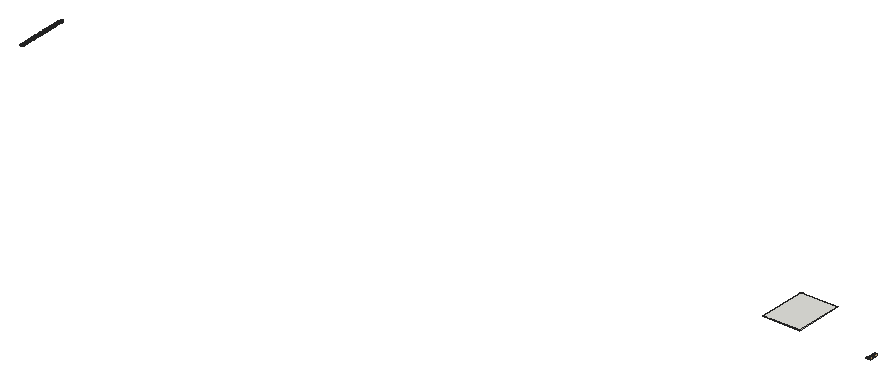
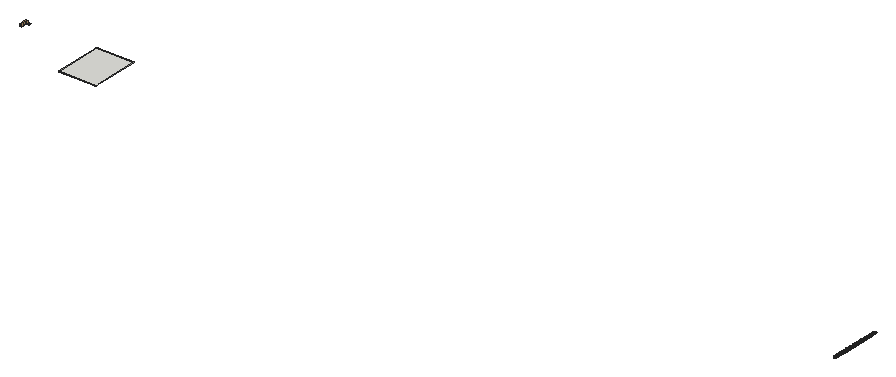
# SketchUp Ruby script. Lengths in inches.
U = 1.inch
M = Sketchup.active_model
def pt(a) = Geom::Point3d.new(a.map { |v| v * U })
def face(e, loops, mat)
  f = e.add_face(loops[0].map { |a| pt(a) })
  loops[1..].each { |l| e.add_face(l.map { |a| pt(a) }).erase! }
  f.material = f.back_material = mat if mat
  f
end
# faces: each face lists its corners as indices into pts; further lists are holes
def faces(e, pts, list, mat = nil) = list.each { |f| face(e, (f[0].is_a?(Array) ? f : [f]).map { |l| l.map { |i| pts[i] } }, mat) }
# xy, xz, yz: faces in a plane at the given z, y or x. An outline is a flat list of corners, or four numbers for a rectangle; further outlines are holes
def ring(l) = l.size == 4 ? [[l[0], l[1]], [l[2], l[1]], [l[2], l[3]], [l[0], l[3]]] : l.each_slice(2).to_a
def flat(e, list, mat, &to3) = list.each { |f| face(e, (f[0].is_a?(Array) ? f : [f]).map { |l| ring(l).map { |u, v| to3.(u, v) } }, mat) }
def xy(e, z, list, mat = nil) = flat(e, list, mat) { |x, y| [x, y, z] }
def xz(e, y, list, mat = nil) = flat(e, list, mat) { |x, z| [x, y, z] }
def yz(e, x, list, mat = nil) = flat(e, list, mat) { |y, z| [x, y, z] }
def lines(e, pts, list) = list.each { |a, b| e.add_line(pt(pts[a]), pt(pts[b])) }
# prism: a flat outline (further loops are holes) pulled along v
def prism(e, loops, v, mat = nil)
  f = face(e, loops, mat); d = Geom::Vector3d.new(v.map { |x| x * U })
  f.pushpull(f.normal.samedirection?(d) ? d.length : -d.length)
end
def box(e, o, s, mat = nil) = prism(e, [[o, [o[0] + s[0], o[1], o[2]], [o[0] + s[0], o[1] + s[1], o[2]], [o[0], o[1] + s[1], o[2]]]], [0, 0, s[2]], mat)
def at(x, y, z, deg = 0) = Geom::Transformation.translation(pt([x, y, z])) * Geom::Transformation.rotation(ORIGIN, Z_AXIS, deg.degrees)
def axes(o, x, y, z) = Geom::Transformation.new([*x, 0, *y, 0, *z, 0, *pt(o).to_a, 1])
def part(name) = M.definitions.add(name)
# library, detail: a bought-in or finely detailed component or shape, given as its bounding box
def library(name, o, s) = part(name).tap { |d| box(d.entities, o, s) }
def detail(e, o, s) = box(e.add_group.entities, o, s)
def put(e, d, t, mat = nil) = e.add_instance(d, t).tap { |i| i.material = mat if mat }
def group(e, t, mat = nil) = e.add_group.tap { |g| g.transformation = t; g.material = mat if mat }.entities
root = M.entities
M.materials.add("Material10").color = [48, 90, 38]
M.materials.add("Material11").color = [68, 110, 48]
M.materials.add("Material12").color = [48, 90, 48]
M.materials.add("Material13").color = [58, 110, 58]
M.materials.add("Material14").color = [58, 90, 38]
M.materials.add("Material15").color = [68, 100, 58]
M.materials.add("Material16").color = [48, 100, 38]
M.materials.add("Material9").color = [68, 110, 58]
c1 = part("grass00")
p = [[-0.6875,0.15,0],[-0.56,0.08,5.52],[-0.04,0.03,2.76],[0.48,-0.02,0],[0.35,-0.02,5.52],[-0.1,-0.14,5.52],
  [-0.12,0.65,8.37],[-0.42,0.65,8.37]]
faces(c1.entities,p,[[0,1,2,3],[3,2,4],[1,5,2],[5,4,2],[1,6,5],[4,5,6],[7,6,1]])
c2 = part("Group16\#1")
put(c2.entities,c1,axes([1.44,-0.61,-0.01],[0.05352,0.12609,0],[-0.10704,0.04543,0.07239],[0.06664,-0.02828,0.11628]),"Material12")
put(c2.entities,c1,axes([0.76,-0.15,-0.01],[0.04676,0.24062,0],[-0.23162,0.04501,0.06642],[0.0652,-0.01267,0.23595]),"Material9")
put(c2.entities,c1,axes([0.79,0.01,-0.01],[-0.00606,0.34651,0],[-0.34381,-0.00602,0.0432],[0.04319,0.00076,0.34386]))
put(c2.entities,c1,axes([1,0.23,-0.01],[-0.07192,0.31144,0],[-0.28722,-0.06632,0.1236],[0.12043,0.02781,0.29478]),"Material11")
put(c2.entities,c1,axes([1.66,0.77,-0.01],[-0.13828,0.29651,0],[-0.21551,-0.1005,0.22471],[0.20365,0.09498,0.23779]),"Material16")
put(c2.entities,c1,axes([0.6875,0.52,-0.01],[-0.18126,0.24051,0],[-0.22746,-0.17142,0.09788],[0.07817,0.05891,0.28481]),"Material11")
put(c2.entities,c1,axes([0.68,0.78,-0.01],[-0.215,0.18688,0],[-0.12385,-0.14248,0.21334],[0.13995,0.16101,0.18878]),"Material9")
put(c2.entities,c1,axes([0.56,1,-0.01],[-0.13756,0.07624,0],[-0.06159,-0.11112,0.0927],[0.04494,0.08108,0.12705]),"Material11")
put(c2.entities,c1,axes([0.2,0.64,-0.01],[-0.23729,0.07254,0],[-0.05711,-0.18681,0.153],[0.04473,0.14632,0.19535]),"Material16")
put(c2.entities,c1,axes([0.0625,0.72,-0.01],[-0.28874,0.02525,0],[-0.02179,-0.24916,0.14647],[0.01276,0.14591,0.25012]),"Material9")
put(c2.entities,c1,axes([-0.08,0.62,-0.01],[-0.34089,-0.04187,0],[0.03255,-0.26504,0.216],[-0.02633,0.21439,0.26703]),"Material16")
put(c2.entities,c1,axes([-0.34,0.98,-0.01],[-0.14314,-0.0493,0],[0.04397,-0.12769,0.06843],[-0.02228,0.0647,0.13505]),"Material16")
put(c2.entities,c1,axes([-0.87,1.45,-0.01],[-0.23488,-0.14114,0],[0.13761,-0.22901,0.06087],[-0.03135,0.05217,0.26717]))
put(c2.entities,c1,axes([-0.72,0.77,-0.01],[-0.14208,-0.13251,0],[0.07209,-0.0773,0.16301],[-0.11118,0.11922,0.1057]),"Material16")
put(c2.entities,c1,axes([-0.62,0.43,-0.01],[-0.14845,-0.21203,0],[0.18654,-0.13061,0.12304],[-0.10079,0.07057,0.22772]),"Material9")
put(c2.entities,c1,axes([-0.68,0.29,-0.01],[-0.13639,-0.32136,0],[0.31723,-0.13464,0.05579],[-0.05136,0.0218,0.34462]),"Material10")
put(c2.entities,c1,axes([-0.64,0.125,-0.01],[-0.0458,-0.23569,0],[0.22124,-0.043,0.08276],[-0.08124,0.01579,0.22538]),"Material13")
put(c2.entities,c1,axes([-1.6,-0.03,-0.01],[0.00576,-0.32897,0],[0.27526,0.00482,0.18018],[-0.18015,-0.00315,0.2753]),"Material11")
put(c2.entities,c1,axes([-1.36,-0.31,-0.01],[0.05718,-0.24765,0],[0.18172,0.04196,0.17267],[-0.16825,-0.03885,0.1865]),"Material16")
put(c2.entities,c1,axes([-1.54,-0.72,-0.01],[0.06537,-0.14017,0],[0.13555,0.06321,0.03939],[-0.0357,-0.01665,0.14956]))
put(c2.entities,c1,axes([-1.19,-0.9,-0.01],[0.09597,-0.12735,0],[0.11214,0.08451,0.07557],[-0.06035,-0.04548,0.14042]),"Material15")
put(c2.entities,c1,axes([-0.47,-0.54,-0.01],[0.11588,-0.10072,0],[0.0618,0.0711,0.12124],[-0.07953,-0.0915,0.0942]))
put(c2.entities,c1,axes([-0.47,-0.84,-0.01],[0.11927,-0.0661,0],[0.06603,0.11913,0.00646],[-0.00313,-0.00565,0.13621]),"Material11")
put(c2.entities,c1,axes([-0.38,-1.24,-0.01],[0.28037,-0.08571,0],[0.0618,0.20215,0.20315],[-0.05939,-0.19428,0.21139]),"Material15")
put(c2.entities,c1,axes([-0.06,-0.66,-0.01],[0.22719,-0.01987,0],[0.01247,0.14255,0.17758],[-0.01547,-0.17691,0.1431]),"Material14")
put(c2.entities,c1,axes([0.11,-0.89,-0.01],[0.14882,0.01828,0],[-0.01058,0.08611,0.12229],[0.01491,-0.12138,0.08676]),"Material12")
put(c2.entities,c1,axes([0.25,-0.72,-0.01],[0.20481,0.07053,0],[-0.06206,0.18022,0.10291],[0.03351,-0.0973,0.1906]),"Material12")
put(c2.entities,c1,axes([0.85,-1.42,-0.01],[0.16481,0.09904,0],[-0.09472,0.15762,0.05616],[0.02893,-0.04814,0.18389]),"Material11")
put(c2.entities,c1,axes([1.01,-1.09,-0.01],[0.21858,0.20385,0],[-0.17495,0.1876,0.15339],[0.10462,-0.11218,0.25652]),"Material16")
put(c2.entities,c1,axes([1.01,-0.71,-0.01],[0.08733,0.12473,0],[-0.06445,0.04512,0.13037],[0.1068,-0.07477,0.07867]),"Material12")
c3 = part("Group15\#1")
put(c3.entities,c2,at(0,0,0))
c4 = part("3darcstudiotree_grass00\#1")
put(c4.entities,c3,at(0,0,0))
c5 = library("J",[-129.92,-126.37,0],[259.84,252.74,0.01])
c6 = library("TR-2",[-11.88,-12.55,0],[23.76,25.1,0.01])
c7 = library("COVER",[-32.47,-52.65,0],[64.94,105.3,0.01])
c8 = library("A$C290B07F5",[-9.78,-10.21,-11.91],[19.56,20.42,23.82])
put(root,c4,axes([958.25,505.875,12.99],[0.09977,6.5925,0],[-2.7746,0.21941,-0.02489],[-0.12601,0.00996,1.9295]))
put(root,c4,axes([959.52,457.8125,12.99],[-3.05412,1.04398,0],[-0.51181,-7.8236,-0.06496],[-0.03818,-0.58357,1.88637]))
put(root,c4,axes([959.125,577.64,12.99],[-1.85992,4.9049,0],[-2.06574,-4.09302,-0.04719],[-0.12383,-0.24536,1.30223]))
put(root,c4,axes([958.92,384.54,12.99],[-1.26269,4.79068,0],[-2.9337,-4.04036,-0.04504],[-0.16016,-0.22058,1.9506]))
put(root,c4,axes([959.68,637.99,12.99],[-3.32889,0.54423,0],[-0.24336,-7.7782,-0.06114],[-0.0162,-0.51767,1.73764]))
put(root,c4,axes([959.72,523.01,12.99],[-3.10393,1.46966,0],[-0.71041,-7.83985,-0.05761],[-0.04177,-0.46097,1.71741]))
put(root,c4,axes([959.06,423.6,12.99],[2.8083,-4.52209,0],[1.62246,5.26481,-0.03692],[0.10104,0.32786,1.83631]))
put(root,c4,axes([959.125,610.9,12.99],[2.37767,-4.57437,0],[1.66372,4.51863,-0.04982],[0.1294,0.35144,1.4295]))
put(root,c4,axes([959.45,648.45,12.99],[-1.8583,6.32941,0],[-2.47729,-3.80045,-0.03945],[-0.12845,-0.19705,1.6047]))
put(root,c4,axes([958.91,411.82,12.99],[1.75279,5.18728,0],[-2.64744,4.67435,-0.04605],[-0.11439,0.20197,1.44046]))
put(root,c4,axes([959.82,348.04,12.99],[1.23043,-4.91559,0],[2.44904,3.2032,-0.04415],[0.19693,0.25757,1.98924]))
put(root,c4,axes([959.36,745.2,12.99],[2.66016,1.99295,0],[-0.98085,6.84099,-0.04711],[-0.05289,0.36892,1.55738]))
put(root,c4,axes([960.61,587.51,12.99],[-2.73686,-2.13189,0],[1.11514,-7.48034,-0.06303],[0.06905,-0.46316,1.61067]))
put(root,c4,axes([960.63,477.56,12.99],[-0.46589,-6.79327,0],[3.44268,-1.23369,-0.06318],[0.18217,-0.06528,1.39517]))
put(root,c4,axes([959.86,545.98,12.99],[-0.25403,6.70401,0],[-2.55694,-0.50626,-0.04948],[-0.19932,-0.03946,1.42361]))
put(root,c4,axes([959.54,569.77,12.99],[1.30406,5.02108,0],[-2.59508,3.52173,-0.05173],[-0.14833,0.20129,1.38038]))
put(root,c4,axes([959.49,354.25,12.99],[1.86626,6.793,0],[-2.60453,3.73892,-0.052],[-0.18537,0.2661,1.7759]))
put(root,c4,axes([960.07,443.3125,12.99],[2.46457,-5.50132,0],[2.19063,5.12801,-0.04175],[0.11016,0.25788,1.62422]))
put(root,c4,axes([960.84,318.93,12.99],[-1.54091,-6.59418,0],[2.84383,-3.47237,-0.05822],[0.22409,-0.27362,1.92982]))
put(root,c4,axes([960.47,727.76,12.99],[1.79923,-6.31413,0],[2.92121,4.34953,-0.04483],[0.13058,0.19442,1.66248]))
put(root,c4,axes([960.2,391.3125,12.99],[0.18223,7.62908,0],[-3.09462,0.38625,-0.05861],[-0.27087,0.03381,1.96776]))
put(root,c4,axes([960.1,552.51,12.99],[3.36894,-0.09386,0],[0.03108,5.82911,-0.04731],[0.00262,0.49102,1.58849]))
put(root,c4,axes([960.1,327.2,12.99],[2.90947,1.59897,0],[-0.81661,7.76412,-0.03506],[-0.02266,0.21549,1.32515]))
put(root,c4,axes([960.86,700.38,12.99],[2.62882,0.25699,0],[-0.13173,7.04108,-0.05798],[-0.0094,0.50235,1.60438]))
put(root,c4,axes([960.66,681.66,12.99],[1.75324,4.67736,0],[-2.61624,5.12418,-0.05975],[-0.13354,0.26155,1.3909]))
put(root,c4,axes([962.89,314.85,12.99],[-1.25433,-7.40959,0],[3.13058,-2.76916,-0.05475],[0.20912,-0.18497,1.88574]))
put(root,c4,axes([963.05,495.47,12.99],[-1.41033,-6.1107,0],[2.57113,-3.10068,-0.03938],[0.12129,-0.14627,1.38871]))
put(root,c4,axes([963.07,601,12.99],[-2.89165,0.00726,0],[-0.00296,-6.17093,-0.04481],[-0.00023,-0.47118,1.70362]))
put(root,c4,axes([962.28,329.85,12.99],[-0.78034,5.83461,0],[-2.89279,-2.02158,-0.0271],[-0.10804,-0.07551,1.72974]))
put(root,c4,axes([963.23,690.32,12.99],[-2.71867,-1.13095,0],[0.48816,-6.13175,-0.02729],[0.02445,-0.30707,1.8715]))
put(root,c4,axes([963.24,298.43,12.99],[-3.00742,2.17634,0],[-0.87057,-6.28606,-0.03323],[-0.04495,-0.3246,1.77353]))
put(root,c4,axes([963.14,704.35,12.99],[0.78767,-7.32748,0],[2.87395,1.61427,-0.05295],[0.25024,0.14056,1.97565]))
put(root,c4,axes([963.47,684.83,12.99],[1.09574,-6.17867,0],[3.21705,2.98109,-0.03495],[0.12513,0.11595,1.83937]))
put(root,c4,axes([962.54,269.98,12.99],[3.14851,0.75939,0],[-0.27317,5.91796,-0.03171],[-0.01598,0.34627,1.71518]))
put(root,c4,axes([963.61,670.62,12.99],[0.35201,-7.72088,0],[2.50173,0.59599,-0.02929],[0.13167,0.03137,1.55926]))
put(root,c4,axes([963.91,517.57,12.99],[-1.03226,-6.13317,0],[2.76859,-2.43482,-0.0371],[0.16696,-0.14683,1.96201]))
put(root,c4,axes([963.93,471.125,12.99],[-1.58125,-5.45324,0],[2.41137,-3.65355,-0.05028],[0.20583,-0.31186,1.94898]))
put(root,c4,axes([963.76,733.35,12.99],[-1.74994,4.01864,0],[-1.73935,-3.95763,-0.04592],[-0.13824,-0.31454,1.42994]))
put(root,c4,axes([963.6,461.0625,12.99],[-1.20888,4.97314,0],[-2.52004,-3.20084,-0.05151],[-0.21687,-0.27546,1.90487]))
put(root,c4,axes([963.1,625.24,12.99],[1.66399,5.54282,0],[-2.2742,3.56741,-0.0512],[-0.15508,0.24327,1.38975]))
put(root,c4,axes([963.61,589.53,12.99],[-1.32159,5.90612,0],[-2.56586,-3.00007,-0.05082],[-0.15474,-0.18093,1.35221]))
put(root,c4,axes([963.07,582.17,12.99],[2.35811,5.77442,0],[-2.27628,4.85722,-0.04297],[-0.14581,0.31113,1.98261]))
put(root,c4,axes([964.07,420.55,12.99],[1.49335,-5.07403,0],[2.78154,4.2776,-0.06298],[0.15147,0.23294,1.33293]))
put(root,c4,axes([964.8,478.96,12.99],[-2.18065,-6.10329,0],[2.63715,-4.92336,-0.03335],[0.10279,-0.19191,1.85855]))
put(root,c4,axes([964.16,605.38,12.99],[-2.58657,4.57339,0],[-1.92231,-5.68088,-0.05181],[-0.10679,-0.3156,1.45196]))
put(root,c4,axes([964.21,657.875,12.99],[0.14502,-7.35383,0],[2.44912,0.25237,-0.03915],[0.2269,0.02338,1.95085]))
put(root,c4,axes([964.375,396.5,12.99],[0.26147,-7.96142,0],[3.43285,0.5891,-0.06273],[0.26073,0.04474,1.9684]))
put(root,c4,axes([964.3125,574.02,12.99],[-2.73578,3.39825,0],[-1.64276,-6.91042,-0.04664],[-0.07711,-0.32437,1.63424]))
put(root,c4,axes([964.22,648.71,12.99],[1.50033,-6.07094,0],[2.6816,3.46281,-0.05349],[0.21692,0.28012,1.96798]))
put(root,c4,axes([964.07,306.37,12.99],[-1.2925,4.85087,0],[-2.37866,-3.31168,-0.03041],[-0.08978,-0.12499,1.3205]))
put(root,c4,axes([963.97,708.34,12.99],[2.84266,-0.11214,0],[0.0543,7.19153,-0.0287],[0.00228,0.30146,1.98369]))
put(root,c4,axes([964.49,348.87,12.99],[2.95484,-1.85365,0],[0.90321,7.52314,-0.05143],[0.04193,0.34927,1.44218]))
put(root,c4,axes([964.84,559.4375,12.99],[2.0751,-5.02262,0],[2.24736,4.85164,-0.05261],[0.12524,0.27038,1.38839]))
put(root,c4,axes([964.46,356.68,12.99],[-0.52284,6.35041,0],[-3.2706,-1.40703,-0.01956],[-0.07636,-0.03285,1.8138]))
put(root,c4,axes([966.29,552.54,12.99],[-0.61527,-5.52026,0],[2.45114,-1.42752,-0.03395],[0.14568,-0.08484,1.53644]))
put(root,c4,axes([966.29,339.01,12.99],[-3.20138,1.77574,0],[-0.82231,-7.74634,-0.06662],[-0.04586,-0.43202,1.39642]))
put(root,c4,axes([966.54,568.08,12.99],[-0.3231,-6.07469,0],[3.42909,-0.953,-0.04217],[0.12494,-0.03472,1.41426]))
put(root,c4,axes([966.68,638.1,12.99],[-2.69493,-1.75469,0],[0.80907,-6.4929,-0.03955],[0.05221,-0.41897,1.95202]))
put(root,c4,axes([966.38,486.68,12.99],[1.04161,-5.03082,0],[2.22394,2.40598,-0.04441],[0.23345,0.25256,1.96303]))
put(root,c4,axes([966.12,592.04,12.99],[2.8708,-1.69734,0],[0.84137,7.43576,-0.04841],[0.04674,0.41305,1.77682]))
put(root,c4,axes([966.3125,663.93,12.99],[2.39899,-2.56372,0],[1.40642,6.87667,-0.04906],[0.08346,0.40806,1.82977]))
put(root,c4,axes([967.19,523.73,12.99],[-0.63258,-6.68651,0],[3.34606,-1.65406,-0.05631],[0.16173,-0.07995,1.37991]))
put(root,c4,axes([966.93,468.34,12.99],[-0.24629,-5.98242,0],[2.56558,-0.55189,-0.04952],[0.18125,-0.03899,1.29958]))
put(root,c4,axes([967.01,449.7,12.99],[-2.61487,4.99382,0],[-1.89279,-5.17874,-0.03098],[-0.07822,-0.21401,1.59479]))
put(root,c4,axes([967.11,428.78,12.99],[-2.2207,3.29662,0],[-1.59231,-5.60472,-0.04277],[-0.10826,-0.38108,1.86401]))
put(root,c4,axes([966.71,307.3125,12.99],[-0.43311,6.76725,0],[-2.54471,-0.851,-0.02144],[-0.11736,-0.03925,1.9513]))
put(root,c4,axes([966.9,422.16,12.99],[2.8975,-3.17759,0],[1.18912,5.66572,-0.04597],[0.08318,0.39632,1.57738]))
put(root,c4,axes([967.99,517.86,12.99],[-2.08888,-3.36158,0],[1.61687,-5.24992,-0.03828],[0.11336,-0.36808,1.98208]))
put(root,c4,axes([967.09,653.42,12.99],[0.11446,7.12574,0],[-3.00644,0.25233,-0.05084],[-0.20964,0.0176,1.70302]))
put(root,c4,axes([967.22,441.23,12.99],[2.41753,-1.1534,0],[0.53932,5.90674,-0.04941],[0.04051,0.44372,1.4533]))
put(root,c4,axes([967.42,681.6875,12.99],[2.33787,-3.83583,0],[1.41774,4.51505,-0.02763],[0.06404,0.20393,1.3256]))
put(root,c4,axes([968.15,648.3,12.99],[-0.93589,-5.29285,0],[2.91557,-2.69378,-0.05241],[0.18838,-0.17405,1.67241]))
put(root,c4,axes([968.26,703.49,12.99],[-2.96957,-0.74013,0],[0.29983,-6.28586,-0.05296],[0.02452,-0.51406,1.62079]))
put(root,c4,axes([968.5,692.72,12.99],[-0.65145,-7.22971,0],[2.7142,-1.27792,-0.02826],[0.11603,-0.05463,1.59374]))
put(root,c4,axes([967.95,710.22,12.99],[-1.69996,5.90717,0],[-2.7999,-4.21024,-0.04701],[-0.13879,-0.20869,1.62457]))
put(root,c4,axes([968.04,277.82,12.99],[-1.60186,5.49601,0],[-2.24418,-3.41774,-0.03773],[-0.12012,-0.18293,1.41517]))
put(root,c4,axes([967.47,457.89,12.99],[2.985,1.87212,0],[-0.79943,6.66037,-0.02738],[-0.03292,0.2743,1.88342]))
put(root,c4,axes([967.87,399.32,12.99],[3.20801,-3.0642,0],[1.34471,7.35619,-0.05614],[0.07111,0.38901,1.57175]))
put(root,c4,axes([968.625,349.38,12.99],[1.43527,-7.20041,0],[2.72682,2.84012,-0.02827],[0.12145,0.12649,1.94019]))
put(root,c4,axes([968.11,374.62,12.99],[0.55766,7.33508,0],[-2.4144,0.95913,-0.03272],[-0.17696,0.0703,1.8454]))
put(root,c4,axes([967.92,384.24,12.99],[2.18024,4.16082,0],[-2.06294,5.64827,-0.05497],[-0.14118,0.38656,1.76958]))
put(root,c4,axes([968.03,558.92,12.99],[2.94736,0.89479,0],[-0.45537,7.83752,-0.05242],[-0.02724,0.46884,1.87281]))
put(root,c4,axes([968.75,319.56,12.99],[1.72286,-5.18057,0],[2.77147,4.81599,-0.05929],[0.14839,0.25785,1.50135]))
put(root,c4,axes([968.68,741.2,12.99],[2.44234,-1.90523,0],[0.82659,5.53674,-0.02189],[0.03747,0.25095,1.86062]))
put(root,c4,axes([968.5625,271.26,12.99],[-0.3749,6.22653,0],[-3.07484,-0.96738,-0.0385],[-0.13941,-0.04386,1.55608]))
put(root,c4,axes([968.77,624.14,12.99],[-0.22422,5.70099,0],[-2.51848,-0.51757,-0.0349],[-0.14201,-0.02918,1.41691]))
put(root,c4,axes([968.82,676.56,12.99],[2.46665,-0.42762,0],[0.23538,7.0944,-0.06006],[0.01628,0.49077,1.53056]))
put(root,c4,axes([968.85,291.32,12.99],[3.15931,-2.58524,0],[1.07102,6.83904,-0.05713],[0.0654,0.41764,1.48067]))
put(root,c4,axes([969.15,747.39,12.99],[1.67238,6.63013,0],[-2.54222,3.35067,-0.02249],[-0.07869,0.10371,1.62577]))
put(root,c4,axes([970.86,404.7,12.99],[-2.50589,-3.50401,0],[1.78731,-6.67882,-0.03935],[0.06297,-0.23529,1.44076]))
put(root,c4,axes([970.49,676.1,12.99],[0.86875,-7.06535,0],[2.97968,1.91441,-0.04021],[0.15825,0.10167,1.73573]))
put(root,c4,axes([970.75,709.94,12.99],[-2.47551,2.72268,0],[-1.32725,-6.30561,-0.05656],[-0.09019,-0.42849,1.54444]))
put(root,c4,axes([970.89,739.93,12.99],[-2.45577,2.72084,0],[-1.0793,-5.09016,-0.04774],[-0.10199,-0.48099,1.66266]))
put(root,c4,axes([971.17,526.05,12.99],[-2.07493,-3.88916,0],[1.70485,-4.75267,-0.04795],[0.11462,-0.31954,1.39039]))
put(root,c4,axes([970.48,539.66,12.99],[2.42509,-2.61535,0],[1.34289,6.50641,-0.02435],[0.04079,0.19763,1.69455]))
put(root,c4,axes([970.83,430.81,12.99],[1.63139,-4.16718,0],[2.03914,4.17126,-0.01984],[0.07176,0.14679,1.82222]))
put(root,c4,axes([971.29,700.13,12.99],[-1.52808,-6.31883,0],[2.19936,-2.77914,-0.04183],[0.15796,-0.1996,1.48723]))
put(root,c4,axes([971.35,604.84,12.99],[-1.06414,-6.95861,0],[2.74745,-2.1954,-0.03865],[0.17713,-0.14154,1.9383]))
put(root,c4,axes([970.39,689.07,12.99],[0.79178,7.05633,0],[-3.00013,1.75902,-0.04684],[-0.1516,0.08889,1.41954]))
put(root,c4,axes([970.69,409.49,12.99],[0.50538,7.36535,0],[-2.5041,0.89779,-0.03929],[-0.21819,0.07823,1.95437]))
put(root,c4,axes([970.51,639.82,12.99],[2.91008,1.4082,0],[-0.56512,6.10214,-0.03259],[-0.02914,0.3146,1.61556]))
put(root,c4,axes([970.51,731.4375,12.99],[2.07072,6.41266,0],[-2.07987,3.50934,-0.03251],[-0.12101,0.20419,1.64081]))
put(root,c4,axes([970.98,382.16,12.99],[-0.21365,7.43732,0],[-2.47409,-0.37138,-0.03425],[-0.1623,-0.02436,1.61497]))
put(root,c4,axes([971.32,300.875,12.99],[-1.74704,4.92813,0],[-2.48483,-4.6028,-0.04128],[-0.1118,-0.20709,1.52936]))
put(root,c4,axes([971.01,319.73,12.99],[2.9951,0.24625,0],[-0.10839,6.88897,-0.02702],[-0.00468,0.29773,1.99535]))
put(root,c4,axes([972.38,555.35,12.99],[-2.31052,-3.2117,0],[1.79834,-6.76006,-0.06276],[0.1028,-0.38643,1.49667]))
put(root,c4,axes([971.18,535.1875,12.99],[2.19987,3.31711,0],[-1.53357,5.31429,-0.03997],[-0.10601,0.36735,1.84008]))
put(root,c4,axes([972.55,568.35,12.99],[-1.71147,-4.09081,0],[2.06886,-4.52269,-0.03327],[0.08018,-0.17529,1.30962]))
put(root,c4,axes([971.74,666.61,12.99],[-0.82193,5.55876,0],[-2.50949,-1.93886,-0.04196],[-0.17753,-0.13716,1.62262]))
put(root,c4,axes([971.4375,423.44,12.99],[1.22279,5.18277,0],[-2.27009,2.79857,-0.03445],[-0.15758,0.19426,1.83855]))
put(root,c4,axes([971.79,628.34,12.99],[-1.27639,4.79606,0],[-2.70673,-3.764,-0.02284],[-0.07386,-0.1027,1.64481]))
put(root,c4,axes([972.69,284.35,12.99],[-2.14975,-3.27479,0],[1.78343,-6.11739,-0.04785],[0.10978,-0.37654,1.82518]))
put(root,c4,axes([972.33,717.8,12.99],[-2.3802,3.32967,0],[-1.58081,-5.90468,-0.04749],[-0.07821,-0.29212,1.3106]))
put(root,c4,axes([972.09,558.43,12.99],[-0.48712,6.61449,0],[-2.85273,-1.09774,-0.04712],[-0.15588,-0.05998,1.33133]))
put(root,c4,axes([972.07,372.97,12.99],[2.83126,0.76755,0],[-0.36878,7.10793,-0.05841],[-0.02088,0.40249,1.30397]))
put(root,c4,axes([972.79,448.1,12.99],[-2.17231,3.84202,0],[-1.72942,-5.10936,-0.04163],[-0.09168,-0.27084,1.39503]))
put(root,c4,axes([972.125,338.35,12.99],[1.62267,5.37397,0],[-2.37489,3.747,-0.02215],[-0.07856,0.12395,1.70619]))
put(root,c4,axes([972.62,268.22,12.99],[0.32036,6.62718,0],[-2.48547,0.62781,-0.03685],[-0.18557,0.04687,1.73767]))
put(root,c4,axes([972.75,514.89,12.99],[2.68974,-3.43151,0],[1.37693,5.63951,-0.03495],[0.08361,0.34245,1.90256]))
put(root,c4,axes([972.71,653.49,12.99],[2.95371,4.14438,0],[-1.38987,5.17589,-0.0354],[-0.0987,0.36754,1.94218]))
put(root,c4,axes([973.05,355.61,12.99],[2.76427,-1.07689,0],[0.43466,5.82992,-0.03176],[0.02791,0.3744,1.85682]))
put(root,c4,axes([974.27,562.1,12.99],[-0.82406,7.22183,0],[-2.85264,-1.70085,-0.04083],[-0.18825,-0.11224,1.92702]))
put(root,c4,axes([974.4,301.96,12.99],[2.78331,-3.55571,0],[1.56147,6.38666,-0.04605],[0.07101,0.29042,1.38783]))
put(root,c4,axes([975.33,288.96,12.99],[-2.03806,-4.16361,0],[1.7518,-4.48061,-0.04195],[0.12074,-0.30882,1.55746]))
put(root,c4,axes([974.28,486.17,12.99],[0.84198,7.10034,0],[-3.01113,1.86576,-0.03421],[-0.14951,0.09264,1.93796]))
put(root,c4,axes([975.03,685.51,12.99],[1.65482,-5.85658,0],[2.73419,4.03683,-0.0579],[0.20138,0.29733,1.84885]))
put(root,c4,axes([975.76,358.65,12.99],[-0.77187,-7.21578,0],[3.26734,-1.82625,-0.03172],[0.0913,-0.05103,1.36741]))
put(root,c4,axes([975.28,616.9,12.99],[-2.44392,3.48779,0],[-1.78811,-6.5469,-0.02972],[-0.05519,-0.20205,1.62371]))
put(root,c4,axes([975.88,396.28,12.99],[-2.12649,-4.67252,0],[1.96634,-4.676,-0.02949],[0.10326,-0.24555,1.96656]))
put(root,c4,axes([974.83,672.92,12.99],[3.33656,-1.65573,0],[0.68831,7.24769,-0.03342],[0.03049,0.32103,1.91382]))
put(root,c4,axes([975.99,419.67,12.99],[-2.18885,-5.95155,0],[2.02567,-3.89277,-0.02964],[0.10215,-0.19631,1.63454]))
put(root,c4,axes([974.8125,348.55,12.99],[2.03591,5.51435,0],[-1.98591,3.83115,-0.05003],[-0.19573,0.3776,1.82479]))
put(root,c4,axes([974.93,375.14,12.99],[1.75048,5.83381,0],[-2.18651,3.42815,-0.03781],[-0.14978,0.23484,1.74723]))
put(root,c4,axes([974.98,496.03,12.99],[3.30482,0.47425,0],[-0.19456,7.08436,-0.04601],[-0.00888,0.32339,1.31249]))
put(root,c4,axes([975.05,380.5,12.99],[0.77275,6.3473,0],[-3.17741,2.0213,-0.02844],[-0.11029,0.07016,1.82107]))
put(root,c4,axes([975.62,468.35,12.99],[-1.7168,6.70479,0],[-2.72308,-3.64334,-0.03733],[-0.11058,-0.14795,1.48568]))
put(root,c4,axes([975.68,362.51,12.99],[2.68437,-4.06019,0],[1.60328,5.53875,-0.03005],[0.07842,0.27091,1.88475]))
put(root,c4,axes([976.4375,544.05,12.99],[-2.69688,-0.25448,0],[0.13917,-7.70651,-0.05407],[0.00811,-0.44931,1.68402]))
put(root,c4,axes([975.37,522.24,12.99],[1.75237,4.05681,0],[-2.42492,5.47323,-0.04002],[-0.11126,0.25112,1.82631]))
put(root,c4,axes([976.87,552.59,12.99],[-3.25102,-0.95552,0],[0.33921,-6.03041,-0.03967],[0.02472,-0.43951,1.78282]))
put(root,c4,axes([976.4,635.7,12.99],[2.20118,-5.62708,0],[2.16823,4.43183,-0.03435],[0.11786,0.2409,1.83666]))
put(root,c4,axes([976.19,436.55,12.99],[-0.90951,7.24895,0],[-2.83687,-1.85985,-0.02925],[-0.09449,-0.06195,1.36051]))
put(root,c4,axes([975.94,460.6,12.99],[1.84917,4.62157,0],[-2.19111,4.58094,-0.03451],[-0.11852,0.24778,1.89576]))
put(root,c4,axes([977.09,582.13,12.99],[-2.85547,0.52305,0],[-0.27378,-7.80988,-0.02116],[-0.00644,-0.18384,1.79229]))
put(root,c4,axes([976.2,305.76,12.99],[3.45801,0.4588,0],[-0.18739,7.37983,-0.0212],[-0.00544,0.21439,1.96575]))
put(root,c4,axes([976.41,428.97,12.99],[2.88154,2.22383,0],[-1.09844,7.4371,-0.0473],[-0.06106,0.41341,1.90097]))
put(root,c4,axes([976.58,336.84,12.99],[2.6804,1.65774,0],[-0.69555,5.87646,-0.04799],[-0.05501,0.46473,1.60328]))
put(root,c4,axes([976.71,652.15,12.99],[0.97179,5.71356,0],[-3.15714,2.80585,-0.01993],[-0.07963,0.07077,1.99239]))
put(root,c4,axes([977.14,591.59,12.99],[3.41546,-1.55281,0],[0.6792,7.80602,-0.02703],[0.01891,0.21729,1.71263]))
put(root,c4,axes([977.24,727.91,12.99],[0.57605,7.47315,0],[-3.17239,1.27775,-0.04576],[-0.16813,0.06772,1.64855]))
put(root,c4,axes([977.12,533.93,12.99],[2.15944,5.74962,0],[-2.18019,4.2786,-0.03135],[-0.10535,0.20674,1.74596]))
put(root,c4,axes([978.42,597.53,12.99],[-3.23171,-0.39368,0],[0.1632,-7.00002,-0.04256],[0.009,-0.38619,1.67228]))
put(root,c4,axes([978.89,562.21,12.99],[-0.4838,-7.03557,0],[3.39795,-1.22094,-0.0381],[0.15419,-0.0554,1.93318]))
put(root,c4,axes([978.87,291.45,12.99],[-2.03152,-3.88207,0],[1.8522,-5.06466,-0.04185],[0.11808,-0.32287,1.7425]))
put(root,c4,axes([978.84,664.5625,12.99],[-2.39926,-3.31217,0],[1.2592,-4.7661,-0.04514],[0.11498,-0.43519,1.64638]))
put(root,c4,axes([979.07,428.64,12.99],[-1.63583,-4.85005,0],[2.42357,-4.27122,-0.03514],[0.11701,-0.20621,1.76492]))
put(root,c4,axes([978.44,540.71,12.99],[2.33503,-3.46517,0],[1.42067,5.00227,-0.02789],[0.07277,0.25624,1.71527]))
put(root,c4,axes([978.65,486.3,12.99],[-1.02252,6.60088,0],[-2.36831,-1.91697,-0.04758],[-0.20503,-0.16596,1.57537]))
put(root,c4,axes([979.42,309.22,12.99],[-3.04407,-2.2839,0],[0.91728,-6.38831,-0.0393],[0.05194,-0.36174,1.71017]))
put(root,c4,axes([978.75,720.55,12.99],[2.22904,-6.15175,0],[1.96837,3.72675,-0.04892],[0.17106,0.32386,1.59182]))
put(root,c4,axes([978.63,497.12,12.99],[-0.09797,7.16444,0],[-2.66376,-0.19034,-0.04056],[-0.15314,-0.01094,1.38085]))
put(root,c4,axes([979.23,738.31,12.99],[-1.35695,5.45247,0],[-2.40866,-3.13222,-0.04597],[-0.13915,-0.18096,1.32398]))
put(root,c4,axes([979.1,747.85,12.99],[2.67753,-2.93476,0],[1.12194,5.34855,-0.03326],[0.06639,0.31651,1.64345]))
put(root,c4,axes([979.39,399.14,12.99],[2.68711,-1.58796,0],[0.77006,6.80886,-0.04398],[0.04925,0.43543,1.88821]))
put(root,c4,axes([979.63,591.67,12.99],[-0.82789,6.54003,0],[-3.2281,-2.13522,-0.06381],[-0.22195,-0.14681,1.66913]))
put(root,c4,axes([979.35,273,12.99],[3.23948,2.28856,0],[-0.99764,7.37894,-0.04987],[-0.05132,0.37957,1.61513]))
g1 = group(root,at(8188.44,514.85,12.75))
box(g1,[0,-1.45,0],[366,477,4])
put(root,c5,axes([9215.76,522.32,0],[-0.00039,-0.04626,0],[-0.04626,0.00039,0],[0,0,0.04626]))
put(root,c5,axes([9225.37,522.45,0],[-0.00039,-0.04626,0],[-0.04626,0.00039,0],[0,0,0.04626]))
put(root,c6,axes([9236.79,524.45,0],[0,0.68156,0],[-0.68156,0,0],[0,0,0.68156]))
put(root,c7,axes([9251.58,535.61,0],[-0.21619,0.06661,0],[-0.06661,-0.21619,0],[0,0,0.22622]))
put(root,c7,axes([9251.58,560.41,0],[-0.21619,0.06661,0],[-0.06661,-0.21619,0],[0,0,0.22622]))
put(root,c7,axes([9251.58,571,0],[-0.21619,0.06661,0],[-0.06661,-0.21619,0],[0,0,0.22622]))
put(root,c8,axes([9251.64,523.89,9.97],[-0.82717,-0.12894,0],[-0.12894,0.82717,0],[0,0,0.83716]))
put(root,c8,axes([9251.64,545.7,9.97],[-0.82717,-0.12894,0],[-0.12894,0.82717,0],[0,0,0.83716]))
put(root,c8,axes([9251.64,556.28,9.97],[-0.82717,-0.12894,0],[-0.12894,0.82717,0],[0,0,0.83716]))
put(root,c8,axes([9251.64,581.89,9.97],[-0.82717,-0.12894,0],[-0.12894,0.82717,0],[0,0,0.83716]))
